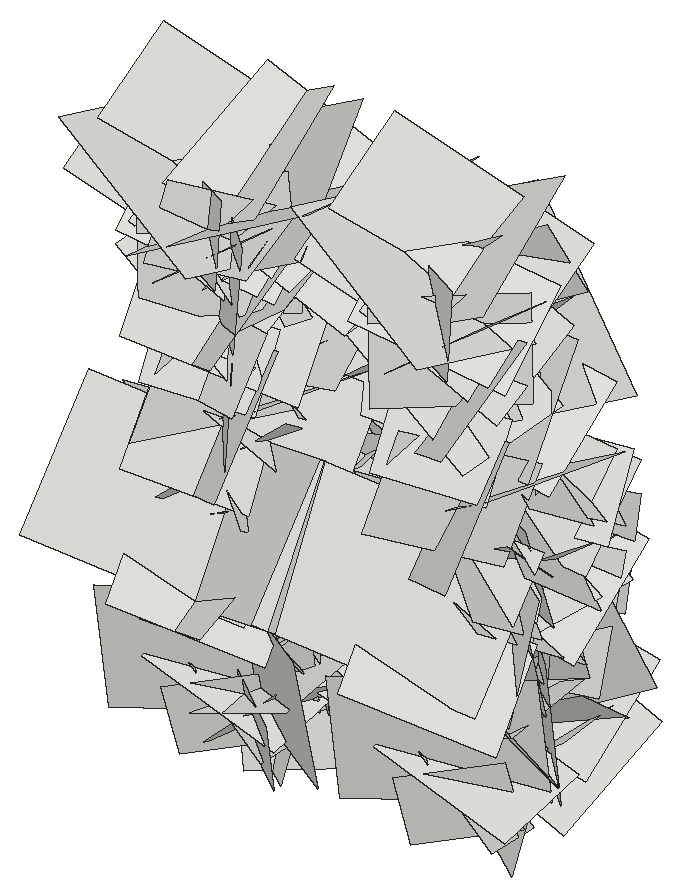
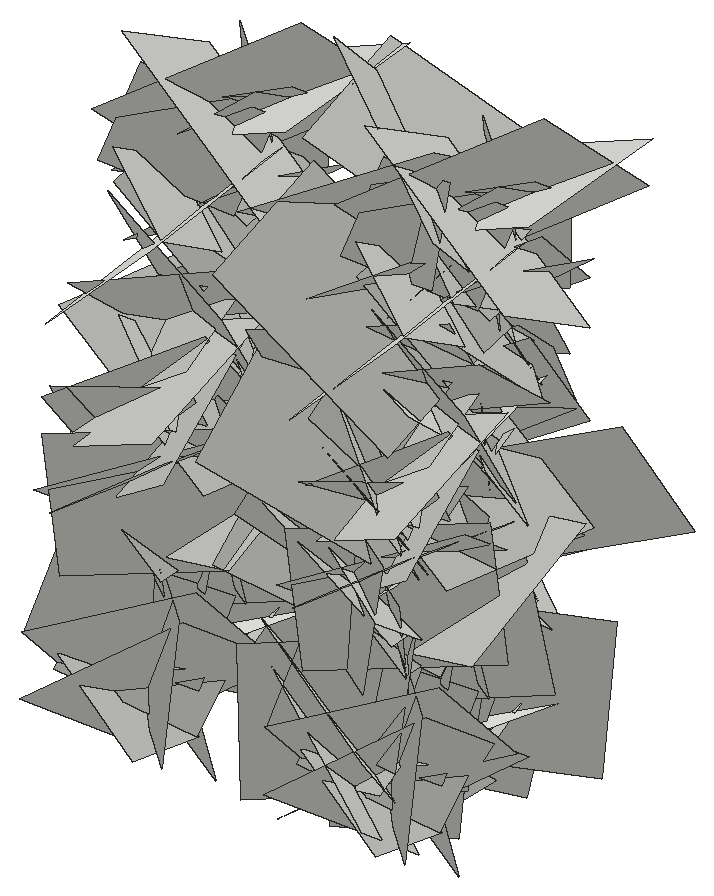
# SketchUp Ruby script. Lengths in inches.
U = 1.inch
M = Sketchup.active_model
def pt(a) = Geom::Point3d.new(a.map { |v| v * U })
def face(e, loops, mat)
  f = e.add_face(loops[0].map { |a| pt(a) })
  loops[1..].each { |l| e.add_face(l.map { |a| pt(a) }).erase! }
  f.material = f.back_material = mat if mat
  f
end
# faces: each face lists its corners as indices into pts; further lists are holes
def faces(e, pts, list, mat = nil) = list.each { |f| face(e, (f[0].is_a?(Array) ? f : [f]).map { |l| l.map { |i| pts[i] } }, mat) }
# xy, xz, yz: faces in a plane at the given z, y or x. An outline is a flat list of corners, or four numbers for a rectangle; further outlines are holes
def ring(l) = l.size == 4 ? [[l[0], l[1]], [l[2], l[1]], [l[2], l[3]], [l[0], l[3]]] : l.each_slice(2).to_a
def flat(e, list, mat, &to3) = list.each { |f| face(e, (f[0].is_a?(Array) ? f : [f]).map { |l| ring(l).map { |u, v| to3.(u, v) } }, mat) }
def xy(e, z, list, mat = nil) = flat(e, list, mat) { |x, y| [x, y, z] }
def xz(e, y, list, mat = nil) = flat(e, list, mat) { |x, z| [x, y, z] }
def yz(e, x, list, mat = nil) = flat(e, list, mat) { |y, z| [x, y, z] }
def lines(e, pts, list) = list.each { |a, b| e.add_line(pt(pts[a]), pt(pts[b])) }
# prism: a flat outline (further loops are holes) pulled along v
def prism(e, loops, v, mat = nil)
  f = face(e, loops, mat); d = Geom::Vector3d.new(v.map { |x| x * U })
  f.pushpull(f.normal.samedirection?(d) ? d.length : -d.length)
end
def box(e, o, s, mat = nil) = prism(e, [[o, [o[0] + s[0], o[1], o[2]], [o[0] + s[0], o[1] + s[1], o[2]], [o[0], o[1] + s[1], o[2]]]], [0, 0, s[2]], mat)
def at(x, y, z, deg = 0) = Geom::Transformation.translation(pt([x, y, z])) * Geom::Transformation.rotation(ORIGIN, Z_AXIS, deg.degrees)
def axes(o, x, y, z) = Geom::Transformation.new([*x, 0, *y, 0, *z, 0, *pt(o).to_a, 1])
def part(name) = M.definitions.add(name)
# library, detail: a bought-in or finely detailed component or shape, given as its bounding box
def library(name, o, s) = part(name).tap { |d| box(d.entities, o, s) }
def detail(e, o, s) = box(e.add_group.entities, o, s)
def put(e, d, t, mat = nil) = e.add_instance(d, t).tap { |i| i.material = mat if mat }
def group(e, t, mat = nil) = e.add_group.tap { |g| g.transformation = t; g.material = mat if mat }.entities
root = M.entities
c1 = part("Component\#6")
p = [[0.01,0,0],[0,3.24,4.54],[4.32,3.24,4.54],[4.33,0,0]]
faces(c1.entities,p,[[0,1,2,3]])
put(root,c1,axes([18.5,177.17,11.87],[-0.09089,-0.73345,-1.16692],[-0.11565,-1.16189,0.73831],[-1.45639,0.13804,0.0142]))
put(root,c1,axes([14.53,177.17,11.87],[0.09089,-0.73345,-1.16692],[0.11565,-1.16189,0.73831],[1.45639,0.13804,0.0142]))
put(root,c1,axes([28.31,177.17,11.87],[-0.09089,-0.73345,-1.16692],[-0.11565,-1.16189,0.73831],[-1.45639,0.13804,0.0142]))
put(root,c1,axes([14.53,171.15,7.72],[-0.19789,0.75168,0.59634],[0.00491,0.60823,-0.76521],[1.01706,0.14332,0.11972]))
put(root,c1,axes([18.5,171.15,7.72],[0.19789,0.75168,0.59634],[-0.00491,0.60823,-0.76521],[-1.01706,0.14332,0.11972]))
put(root,c1,axes([24.34,171.15,7.72],[-0.19789,0.75168,0.59634],[0.00491,0.60823,-0.76521],[1.01706,0.14332,0.11972]))
put(root,c1,axes([14.53,175.79,22.11],[0.09057,-0.18477,-0.67682],[-0.07729,-0.68047,0.17656],[0.73966,-0.04848,0.10132]))
put(root,c1,axes([18.5,175.79,22.11],[-0.09057,-0.18477,-0.67682],[0.07729,-0.68047,0.17656],[-0.73966,-0.04848,0.10132]))
put(root,c1,axes([24.34,175.79,22.11],[0.09057,-0.18477,-0.67682],[-0.07729,-0.68047,0.17656],[0.73966,-0.04848,0.10132]))
put(root,c1,axes([14.53,172.87,15.39],[-0.04258,0.36909,0.59744],[0.18529,0.58484,-0.34955],[0.72096,-0.1285,0.12512]))
put(root,c1,axes([18.5,172.87,15.39],[0.04258,0.36909,0.59744],[-0.18529,0.58484,-0.34955],[-0.72096,-0.1285,0.12512]))
put(root,c1,axes([24.34,172.87,15.39],[-0.04258,0.36909,0.59744],[0.18529,0.58484,-0.34955],[0.72096,-0.1285,0.12512]))
put(root,c1,axes([18.5,176.71,20],[-0.1716,-1.2405,0.25629],[-0.15029,0.2745,1.23906],[-1.33426,0.12862,-0.17253]))
put(root,c1,axes([14.53,176.71,20],[0.1716,-1.2405,0.25629],[0.15029,0.2745,1.23906],[1.33426,0.12862,-0.17253]))
put(root,c1,axes([28.31,176.71,20],[-0.1716,-1.2405,0.25629],[-0.15029,0.2745,1.23906],[-1.33426,0.12862,-0.17253]))
put(root,c1,axes([14.53,172.9,17.79],[-0.05847,0.04666,0.93522],[-0.13105,0.92828,-0.05361],[0.98388,0.12642,0.04844]))
put(root,c1,axes([18.5,172.9,17.79],[0.05847,0.04666,0.93522],[0.13105,0.92828,-0.05361],[-0.98388,0.12642,0.04844]))
put(root,c1,axes([24.34,172.9,17.79],[-0.05847,0.04666,0.93522],[-0.13105,0.92828,-0.05361],[0.98388,0.12642,0.04844]))
put(root,c1,axes([14.53,172.44,13.26],[0.14239,0.27787,0.83247],[-0.25689,0.82117,-0.23499],[0.89411,0.19168,-0.20009]))
put(root,c1,axes([18.5,172.44,13.26],[-0.14239,0.27787,0.83247],[0.25689,0.82117,-0.23499],[-0.89411,0.19168,-0.20009]))
put(root,c1,axes([24.34,172.44,13.26],[0.14239,0.27787,0.83247],[-0.25689,0.82117,-0.23499],[0.89411,0.19168,-0.20009]))
put(root,c1,axes([14.53,178.76,18.36],[-0.19902,-0.79911,-0.76231],[-0.1591,-0.74761,0.82067],[1.1598,-0.23968,-0.01823]))
put(root,c1,axes([18.5,178.76,18.36],[0.19902,-0.79911,-0.76231],[0.1591,-0.74761,0.82067],[-1.1598,-0.23968,-0.01823]))
put(root,c1,axes([24.34,178.76,18.36],[-0.19902,-0.79911,-0.76231],[-0.1591,-0.74761,0.82067],[1.1598,-0.23968,-0.01823]))
put(root,c1,axes([18.5,178.02,21.625],[0.10055,-0.80704,-0.57155],[-0.14009,-0.57937,0.79615],[-1.03886,0.00001,-0.16268]))
put(root,c1,axes([14.53,178.02,21.625],[-0.10055,-0.80704,-0.57155],[0.14009,-0.57937,0.79615],[1.03886,0.00001,-0.16268]))
put(root,c1,axes([28.31,178.02,21.625],[0.10055,-0.80704,-0.57155],[-0.14009,-0.57937,0.79615],[-1.03886,0.00001,-0.16268]))
put(root,c1,axes([18.5,171.875,12.53],[0.03767,0.74177,1.03266],[0.14299,1.02503,-0.74093],[-1.34014,0.13022,-0.05004]))
put(root,c1,axes([14.53,171.875,12.53],[-0.03767,0.74177,1.03266],[-0.14299,1.02503,-0.74093],[1.34014,0.13022,-0.05004]))
put(root,c1,axes([28.31,171.875,12.53],[0.03767,0.74177,1.03266],[0.14299,1.02503,-0.74093],[-1.34014,0.13022,-0.05004]))
put(root,c1,axes([14.53,176.92,18.36],[0.03591,-0.7978,0.13647],[-0.05211,0.13431,0.79737],[0.85636,0.04162,0.0428]))
put(root,c1,axes([18.5,176.92,18.36],[-0.03591,-0.7978,0.13647],[0.05211,0.13431,0.79737],[-0.85636,0.04162,0.0428]))
put(root,c1,axes([24.34,176.92,18.36],[0.03591,-0.7978,0.13647],[-0.05211,0.13431,0.79737],[0.85636,0.04162,0.0428]))
put(root,c1,axes([18.5,176.79,7.17],[-0.05072,0.23896,-1.1979],[-0.10512,-1.19562,-0.23454],[-1.29052,0.088,0.06618]))
put(root,c1,axes([14.53,176.79,7.17],[0.05072,0.23896,-1.1979],[0.10512,-1.19562,-0.23454],[1.29052,0.088,0.06618]))
put(root,c1,axes([28.31,176.79,7.17],[-0.05072,0.23896,-1.1979],[-0.10512,-1.19562,-0.23454],[-1.29052,0.088,0.06618]))
put(root,c1,axes([14.53,175.07,0.3],[-0.05353,-0.16234,0.63718],[-0.01427,0.63917,0.16178],[0.69684,0.00062,0.05226]))
put(root,c1,axes([18.5,175.07,0.3],[0.05353,-0.16234,0.63718],[0.01427,0.63917,0.16178],[-0.69684,0.00062,0.05226]))
put(root,c1,axes([24.34,175.07,0.3],[-0.05353,-0.16234,0.63718],[-0.01427,0.63917,0.16178],[0.69684,0.00062,0.05226]))
put(root,c1,axes([18.5,178.16,17.01],[-0.17232,-1.0163,-0.23365],[0.0611,-0.24487,1.02499],[-1.10369,0.14512,0.09322]))
put(root,c1,axes([14.53,178.16,17.01],[0.17232,-1.0163,-0.23365],[-0.0611,-0.24487,1.02499],[1.10369,0.14512,0.09322]))
put(root,c1,axes([28.31,178.16,17.01],[-0.17232,-1.0163,-0.23365],[0.0611,-0.24487,1.02499],[-1.10369,0.14512,0.09322]))
put(root,c1,axes([18.5,178.75,19.8],[-0.0392,-0.90326,-0.49419],[0.16181,-0.49385,0.89122],[-1.07932,-0.04123,0.15156]))
put(root,c1,axes([14.53,178.75,19.8],[0.0392,-0.90326,-0.49419],[-0.16181,-0.49385,0.89122],[1.07932,-0.04123,0.15156]))
put(root,c1,axes([28.31,178.75,19.8],[-0.0392,-0.90326,-0.49419],[0.16181,-0.49385,0.89122],[-1.07932,-0.04123,0.15156]))
put(root,c1,axes([14.53,174.43,8.39],[-0.03188,0.26889,0.69876],[0.00311,0.69936,-0.269],[0.79363,0.00806,0.02912]))
put(root,c1,axes([18.5,174.43,8.39],[0.03188,0.26889,0.69876],[-0.00311,0.69936,-0.269],[-0.79363,0.00806,0.02912]))
put(root,c1,axes([24.34,174.43,8.39],[-0.03188,0.26889,0.69876],[0.00311,0.69936,-0.269],[0.79363,0.00806,0.02912]))
put(root,c1,axes([18.5,179.79,22.45],[-0.18749,-0.99323,-0.93091],[0.09936,-0.94539,0.99088],[-1.43954,0.06411,0.18963]))
put(root,c1,axes([14.53,179.79,22.45],[0.18749,-0.99323,-0.93091],[-0.09936,-0.94539,0.99088],[1.43954,0.06411,0.18963]))
put(root,c1,axes([28.31,179.79,22.45],[-0.18749,-0.99323,-0.93091],[0.09936,-0.94539,0.99088],[-1.43954,0.06411,0.18963]))
put(root,c1,axes([18.5,177.03,8.61],[-0.03763,-0.79919,0.49947],[0.19388,0.48448,0.78821],[-0.97999,0.12653,0.13676]))
put(root,c1,axes([14.53,177.03,8.61],[0.03763,-0.79919,0.49947],[-0.19388,0.48448,0.78821],[0.97999,0.12653,0.13676]))
put(root,c1,axes([28.31,177.03,8.61],[-0.03763,-0.79919,0.49947],[0.19388,0.48448,0.78821],[-0.97999,0.12653,0.13676]))
put(root,c1,axes([14.53,177.03,9.04],[-0.05145,-0.49737,0.47013],[0.11624,0.45957,0.49752],[0.71609,-0.11034,-0.04698]))
put(root,c1,axes([18.5,177.03,9.04],[0.05145,-0.49737,0.47013],[-0.11624,0.45957,0.49752],[-0.71609,-0.11034,-0.04698]))
put(root,c1,axes([24.34,177.03,9.04],[-0.05145,-0.49737,0.47013],[0.11624,0.45957,0.49752],[0.71609,-0.11034,-0.04698]))
put(root,c1,axes([18.5,179.02,2.63],[0.02304,-0.93672,-0.18796],[-0.20199,-0.18848,0.91728],[-0.99236,0.01662,-0.19107]))
put(root,c1,axes([14.53,179.02,2.63],[-0.02304,-0.93672,-0.18796],[0.20199,-0.18848,0.91728],[0.99236,0.01662,-0.19107]))
put(root,c1,axes([28.31,179.02,2.63],[0.02304,-0.93672,-0.18796],[-0.20199,-0.18848,0.91728],[-0.99236,0.01662,-0.19107]))
put(root,c1,axes([14.53,175.31,3.87],[-0.17194,0.72285,-0.14796],[-0.1038,-0.17124,-0.72925],[0.77519,0.1374,-0.13047]))
put(root,c1,axes([18.5,175.31,3.87],[0.17194,0.72285,-0.14796],[0.1038,-0.17124,-0.72925],[-0.77519,0.1374,-0.13047]))
put(root,c1,axes([24.34,175.31,3.87],[-0.17194,0.72285,-0.14796],[-0.1038,-0.17124,-0.72925],[0.77519,0.1374,-0.13047]))
put(root,c1,axes([18.5,173.88,22.27],[-0.13701,1.18016,0.66561],[-0.07419,0.66193,-1.18721],[-1.4343,-0.14697,-0.00217]))
put(root,c1,axes([14.53,173.88,22.27],[0.13701,1.18016,0.66561],[0.07419,0.66193,-1.18721],[1.4343,-0.14697,-0.00217]))
put(root,c1,axes([28.31,173.88,22.27],[-0.13701,1.18016,0.66561],[-0.07419,0.66193,-1.18721],[-1.4343,-0.14697,-0.00217]))
put(root,c1,axes([18.5,175.28,5.97],[0.1544,0.17587,1.10387],[-0.02973,1.11343,-0.17369],[-1.18449,-0.00502,0.14825]))
put(root,c1,axes([14.53,175.28,5.97],[-0.1544,0.17587,1.10387],[0.02973,1.11343,-0.17369],[1.18449,-0.00502,0.14825]))
put(root,c1,axes([28.31,175.28,5.97],[0.1544,0.17587,1.10387],[-0.02973,1.11343,-0.17369],[-1.18449,-0.00502,0.14825]))
put(root,c1,axes([18.5,174.05,15.13],[0.29087,1.34123,-0.04275],[-0.1118,-0.02194,-1.36543],[-1.41802,0.27684,0.09888]))
put(root,c1,axes([14.53,174.05,15.13],[-0.29087,1.34123,-0.04275],[0.1118,-0.02194,-1.36543],[1.41802,0.27684,0.09888]))
put(root,c1,axes([28.31,174.05,15.13],[0.29087,1.34123,-0.04275],[-0.1118,-0.02194,-1.36543],[-1.41802,0.27684,0.09888]))
put(root,c1,axes([18.5,177.91,2.6],[-0.0759,-0.493,0.60539],[-0.11612,0.60826,0.48238],[-0.8194,-0.04053,-0.12444]))
put(root,c1,axes([14.53,177.91,2.6],[0.0759,-0.493,0.60539],[0.11612,0.60826,0.48238],[0.8194,-0.04053,-0.12444]))
put(root,c1,axes([28.31,177.91,2.6],[-0.0759,-0.493,0.60539],[-0.11612,0.60826,0.48238],[-0.8194,-0.04053,-0.12444]))
put(root,c1,axes([14.53,179.07,16.9375],[0.01654,-0.76992,0.15337],[-0.18248,0.14631,0.752],[0.8119,0.04857,0.16589]))
put(root,c1,axes([18.5,179.07,16.9375],[-0.01654,-0.76992,0.15337],[0.18248,0.14631,0.752],[-0.8119,0.04857,0.16589]))
put(root,c1,axes([24.34,179.07,16.9375],[0.01654,-0.76992,0.15337],[-0.18248,0.14631,0.752],[0.8119,0.04857,0.16589]))
put(root,c1,axes([18.5,177.25,5.58],[-0.00826,-0.19404,0.73725],[-0.12542,0.72866,0.19053],[-0.79831,-0.11247,-0.03756]))
put(root,c1,axes([14.53,177.25,5.58],[0.00826,-0.19404,0.73725],[0.12542,0.72866,0.19053],[0.79831,-0.11247,-0.03756]))
put(root,c1,axes([28.31,177.25,5.58],[-0.00826,-0.19404,0.73725],[-0.12542,0.72866,0.19053],[-0.79831,-0.11247,-0.03756]))
put(root,c1,axes([14.53,178.9,4.98],[-0.12785,-0.58421,0.25103],[0.01096,0.25367,0.59532],[0.67392,-0.11496,0.03794]))
put(root,c1,axes([18.5,178.9,4.98],[0.12785,-0.58421,0.25103],[-0.01096,0.25367,0.59532],[-0.67392,-0.11496,0.03794]))
put(root,c1,axes([24.34,178.9,4.98],[-0.12785,-0.58421,0.25103],[0.01096,0.25367,0.59532],[0.67392,-0.11496,0.03794]))
put(root,c1,axes([14.53,177.55,19],[-0.11507,-0.3549,0.71119],[-0.00206,0.71791,0.35796],[0.84251,-0.04671,0.09801]))
put(root,c1,axes([18.5,177.55,19],[0.11507,-0.3549,0.71119],[0.00206,0.71791,0.35796],[-0.84251,-0.04671,0.09801]))
put(root,c1,axes([24.34,177.55,19],[-0.11507,-0.3549,0.71119],[-0.00206,0.71791,0.35796],[0.84251,-0.04671,0.09801]))
put(root,c1,axes([18.5,179.43,6.59],[-0.14458,-1.15784,0.73248],[-0.20973,0.74503,1.14083],[-1.43706,0.00775,-0.24019]))
put(root,c1,axes([14.53,179.43,6.59],[0.14458,-1.15784,0.73248],[0.20973,0.74503,1.14083],[1.43706,0.00775,-0.24019]))
put(root,c1,axes([28.31,179.43,6.59],[-0.14458,-1.15784,0.73248],[-0.20973,0.74503,1.14083],[-1.43706,0.00775,-0.24019]))
put(root,c1,axes([18.5,177.67,8.79],[-0.10774,-0.22129,0.90038],[-0.20078,0.89162,0.19775],[-0.96207,-0.1613,-0.1421]))
put(root,c1,axes([14.53,177.67,8.79],[0.10774,-0.22129,0.90038],[0.20078,0.89162,0.19775],[0.96207,-0.1613,-0.1421]))
put(root,c1,axes([28.31,177.67,8.79],[-0.10774,-0.22129,0.90038],[-0.20078,0.89162,0.19775],[-0.96207,-0.1613,-0.1421]))
put(root,c1,axes([14.53,179.66,2.51],[-0.14219,-0.09473,-0.68692],[0.01318,-0.69988,0.09409],[0.73491,-0.00578,-0.13459]))
put(root,c1,axes([18.5,179.66,2.51],[0.14219,-0.09473,-0.68692],[-0.01318,-0.69988,0.09409],[-0.73491,-0.00578,-0.13459]))
put(root,c1,axes([24.34,179.66,2.51],[-0.14219,-0.09473,-0.68692],[0.01318,-0.69988,0.09409],[0.73491,-0.00578,-0.13459]))
put(root,c1,axes([14.53,180.59,3.91],[-0.10883,-0.74668,-0.23347],[0.0349,-0.23939,0.75113],[0.82853,-0.08799,-0.06231]))
put(root,c1,axes([18.5,180.59,3.91],[0.10883,-0.74668,-0.23347],[-0.0349,-0.23939,0.75113],[-0.82853,-0.08799,-0.06231]))
put(root,c1,axes([24.34,180.59,3.91],[-0.10883,-0.74668,-0.23347],[0.0349,-0.23939,0.75113],[0.82853,-0.08799,-0.06231]))
put(root,c1,axes([14.53,180.83,12.7],[-0.12371,-0.65209,-0.45157],[-0.04757,-0.45027,0.66181],[0.83942,-0.12162,-0.02905]))
put(root,c1,axes([18.5,180.83,12.7],[0.12371,-0.65209,-0.45157],[0.04757,-0.45027,0.66181],[-0.83942,-0.12162,-0.02905]))
put(root,c1,axes([24.34,180.83,12.7],[-0.12371,-0.65209,-0.45157],[-0.04757,-0.45027,0.66181],[0.83942,-0.12162,-0.02905]))
put(root,c1,axes([18.5,180.99,16.6875],[-0.01817,-0.80344,-0.66577],[-0.22863,-0.64876,0.78846],[-1.08217,0.15055,-0.1554]))
put(root,c1,axes([14.53,180.99,16.6875],[0.01817,-0.80344,-0.66577],[0.22863,-0.64876,0.78846],[1.08217,0.15055,-0.1554]))
put(root,c1,axes([28.31,180.99,16.6875],[-0.01817,-0.80344,-0.66577],[-0.22863,-0.64876,0.78846],[-1.08217,0.15055,-0.1554]))
put(root,c1,axes([18.5,176.29,14.82],[-0.00549,0.62123,1.00169],[-0.24363,0.98194,-0.61017],[-1.22543,-0.19801,0.11682]))
put(root,c1,axes([14.53,176.29,14.82],[0.00549,0.62123,1.00169],[0.24363,0.98194,-0.61017],[1.22543,-0.19801,0.11682]))
put(root,c1,axes([28.31,176.29,14.82],[-0.00549,0.62123,1.00169],[-0.24363,0.98194,-0.61017],[-1.22543,-0.19801,0.11682]))
put(root,c1,axes([14.53,178.54,4.68],[0.06155,-0.26232,0.60589],[0.0363,0.6086,0.26022],[0.69891,-0.00851,-0.06687]))
put(root,c1,axes([18.5,178.54,4.68],[-0.06155,-0.26232,0.60589],[-0.0363,0.6086,0.26022],[-0.69891,-0.00851,-0.06687]))
put(root,c1,axes([24.34,178.54,4.68],[0.06155,-0.26232,0.60589],[0.0363,0.6086,0.26022],[0.69891,-0.00851,-0.06687]))
put(root,c1,axes([18.5,179.8125,11.71],[-0.00414,-0.7832,0.49624],[0.01003,0.49619,0.78318],[-0.98275,0.00836,0.0059]))
put(root,c1,axes([28.31,179.8125,11.71],[-0.00414,-0.7832,0.49624],[0.01003,0.49619,0.78318],[-0.98275,0.00836,0.0059]))
put(root,c1,axes([14.53,179.8125,11.71],[0.00414,-0.7832,0.49624],[-0.01003,0.49619,0.78318],[0.98275,0.00836,0.0059]))
put(root,c1,axes([18.5,181.49,10.05],[-0.07357,-0.24485,-1.22332],[-0.09578,-1.221,0.24951],[-1.31896,0.10233,0.05011]))
put(root,c1,axes([14.53,181.49,10.05],[0.07357,-0.24485,-1.22332],[0.09578,-1.221,0.24951],[1.31896,0.10233,0.05011]))
put(root,c1,axes([28.31,181.49,10.05],[-0.07357,-0.24485,-1.22332],[-0.09578,-1.221,0.24951],[-1.31896,0.10233,0.05011]))
put(root,c1,axes([14.53,181.21,19.66],[-0.0984,-0.57654,-0.29954],[-0.01889,-0.30021,0.58335],[0.68843,-0.09064,-0.02681]))
put(root,c1,axes([18.5,181.21,19.66],[0.0984,-0.57654,-0.29954],[0.01889,-0.30021,0.58335],[-0.68843,-0.09064,-0.02681]))
put(root,c1,axes([24.34,181.21,19.66],[-0.0984,-0.57654,-0.29954],[-0.01889,-0.30021,0.58335],[0.68843,-0.09064,-0.02681]))
put(root,c1,axes([14.53,181.24,7.39],[-0.09835,-0.8461,0.11424],[-0.10744,0.12502,0.84359],[0.89861,-0.07766,0.11336]))
put(root,c1,axes([18.5,181.24,7.39],[0.09835,-0.8461,0.11424],[0.10744,0.12502,0.84359],[-0.89861,-0.07766,0.11336]))
put(root,c1,axes([24.34,181.24,7.39],[-0.09835,-0.8461,0.11424],[-0.10744,0.12502,0.84359],[0.89861,-0.07766,0.11336]))
put(root,c1,axes([18.5,180.26,8.26],[0.04265,-1.00211,0.75475],[0.17142,0.75298,0.99114],[-1.31872,0.06547,0.15325]))
put(root,c1,axes([14.53,180.26,8.26],[-0.04265,-1.00211,0.75475],[-0.17142,0.75298,0.99114],[1.31872,0.06547,0.15325]))
put(root,c1,axes([28.31,180.26,8.26],[0.04265,-1.00211,0.75475],[0.17142,0.75298,0.99114],[-1.31872,0.06547,0.15325]))
put(root,c1,axes([18.5,182.69,9.96],[0.0402,-0.96504,-0.67279],[-0.04089,-0.67379,0.96431],[-1.24632,-0.00902,-0.05333]))
put(root,c1,axes([14.53,182.69,9.96],[-0.0402,-0.96504,-0.67279],[0.04089,-0.67379,0.96431],[1.24632,-0.00902,-0.05333]))
put(root,c1,axes([28.31,182.69,9.96],[0.0402,-0.96504,-0.67279],[-0.04089,-0.67379,0.96431],[-1.24632,-0.00902,-0.05333]))
put(root,c1,axes([18.5,182.3,13.14],[-0.06012,-0.59744,-0.78978],[0.12867,-0.78931,0.58836],[-1.0418,-0.06301,0.11824]))
put(root,c1,axes([14.53,182.3,13.14],[0.06012,-0.59744,-0.78978],[-0.12867,-0.78931,0.58836],[1.0418,-0.06301,0.11824]))
put(root,c1,axes([28.31,182.3,13.14],[-0.06012,-0.59744,-0.78978],[0.12867,-0.78931,0.58836],[-1.0418,-0.06301,0.11824]))
put(root,c1,axes([14.53,181.23,7.68],[0.09173,-0.20092,-0.6203],[-0.07215,-0.6251,0.19298],[0.68737,-0.0388,0.10304]))
put(root,c1,axes([18.5,181.23,7.68],[-0.09173,-0.20092,-0.6203],[0.07215,-0.6251,0.19298],[-0.68737,-0.0388,0.10304]))
put(root,c1,axes([24.34,181.23,7.68],[0.09173,-0.20092,-0.6203],[-0.07215,-0.6251,0.19298],[0.68737,-0.0388,0.10304]))
put(root,c1,axes([18.5,179.12,5.58],[-0.07323,0.67973,-0.51678],[-0.08286,-0.52133,-0.67526],[-0.90131,-0.0073,0.10406]))
put(root,c1,axes([14.53,179.12,5.58],[0.07323,0.67973,-0.51678],[0.08286,-0.52133,-0.67526],[0.90131,-0.0073,0.10406]))
put(root,c1,axes([28.31,179.12,5.58],[-0.07323,0.67973,-0.51678],[-0.08286,-0.52133,-0.67526],[-0.90131,-0.0073,0.10406]))
put(root,c1,axes([18.5,181.89,8.77],[-0.15486,-1.04414,-0.08659],[0.04063,-0.0927,1.0531],[-1.10985,0.1423,0.05063]))
put(root,c1,axes([14.53,181.89,8.77],[0.15486,-1.04414,-0.08659],[-0.04063,-0.0927,1.0531],[1.10985,0.1423,0.05063]))
put(root,c1,axes([28.31,181.89,8.77],[-0.15486,-1.04414,-0.08659],[0.04063,-0.0927,1.0531],[-1.10985,0.1423,0.05063]))
put(root,c1,axes([18.5,182.08,15.67],[-0.13861,-1.35642,0.31459],[0.2886,0.28497,1.34186],[-1.44748,0.1867,0.23742]))
put(root,c1,axes([14.53,182.08,15.67],[0.13861,-1.35642,0.31459],[-0.2886,0.28497,1.34186],[1.44748,0.1867,0.23742]))
put(root,c1,axes([28.31,182.08,15.67],[-0.13861,-1.35642,0.31459],[0.2886,0.28497,1.34186],[-1.44748,0.1867,0.23742]))
put(root,c1,axes([18.5,180.69,8.55],[0.12889,0.40226,-0.91097],[0.04748,-0.91901,-0.39983],[-1.05451,0.00779,-0.12935]))
put(root,c1,axes([28.31,180.69,8.55],[0.12889,0.40226,-0.91097],[0.04748,-0.91901,-0.39983],[-1.05451,0.00779,-0.12935]))
put(root,c1,axes([14.53,180.69,8.55],[-0.12889,0.40226,-0.91097],[-0.04748,-0.91901,-0.39983],[1.05451,0.00779,-0.12935]))
put(root,c1,axes([18.5,178.03,1.86],[-0.09591,-0.07879,1.2407],[0.19288,1.22975,0.09137],[-1.3036,0.18775,-0.07776]))
put(root,c1,axes([14.53,178.03,1.86],[0.09591,-0.07879,1.2407],[-0.19288,1.22975,0.09137],[1.3036,0.18775,-0.07776]))
put(root,c1,axes([28.31,178.03,1.86],[-0.09591,-0.07879,1.2407],[0.19288,1.22975,0.09137],[-1.3036,0.18775,-0.07776]))
put(root,c1,axes([14.53,178.57,11.38],[-0.09025,0.42259,0.64735],[0.15778,0.64804,-0.40347],[0.80413,-0.07973,0.15182]))
put(root,c1,axes([18.5,178.57,11.38],[0.09025,0.42259,0.64735],[-0.15778,0.64804,-0.40347],[-0.80413,-0.07973,0.15182]))
put(root,c1,axes([24.34,178.57,11.38],[-0.09025,0.42259,0.64735],[0.15778,0.64804,-0.40347],[0.80413,-0.07973,0.15182]))
put(root,c1,axes([18.5,181.48,10.98],[-0.16941,-1.10786,0.62997],[0.04307,0.63015,1.11849],[-1.35023,0.1591,-0.04336]))
put(root,c1,axes([14.53,181.48,10.98],[0.16941,-1.10786,0.62997],[-0.04307,0.63015,1.11849],[1.35023,0.1591,-0.04336]))
put(root,c1,axes([28.31,181.48,10.98],[-0.16941,-1.10786,0.62997],[0.04307,0.63015,1.11849],[-1.35023,0.1591,-0.04336]))
put(root,c1,axes([18.5,183.39,2.71],[-0.21072,-0.93049,-0.66529],[0.0846,-0.6849,0.93407],[-1.20954,0.1142,0.18123]))
put(root,c1,axes([14.53,183.39,2.71],[0.21072,-0.93049,-0.66529],[-0.0846,-0.6849,0.93407],[1.20954,0.1142,0.18123]))
put(root,c1,axes([28.31,183.39,2.71],[-0.21072,-0.93049,-0.66529],[0.0846,-0.6849,0.93407],[-1.20954,0.1142,0.18123]))
put(root,c1,axes([18.5,182.3,11.84],[-0.17648,0.01407,-1.1199],[-0.09677,-1.12861,-0.00061],[-1.18323,0.09021,0.16708]))
put(root,c1,axes([14.53,182.3,11.84],[0.17648,0.01407,-1.1199],[0.09677,-1.12861,-0.00061],[1.18323,0.09021,0.16708]))
put(root,c1,axes([28.31,182.3,11.84],[-0.17648,0.01407,-1.1199],[-0.09677,-1.12861,-0.00061],[-1.18323,0.09021,0.16708]))
put(root,c1,axes([18.5,183.3125,5.12],[-0.15127,-0.71846,-0.81538],[-0.11003,-0.80961,0.73154],[-1.14669,0.17246,0.03737]))
put(root,c1,axes([14.53,183.3125,5.12],[0.15127,-0.71846,-0.81538],[0.11003,-0.80961,0.73154],[1.14669,0.17246,0.03737]))
put(root,c1,axes([28.31,183.3125,5.12],[-0.15127,-0.71846,-0.81538],[-0.11003,-0.80961,0.73154],[-1.14669,0.17246,0.03737]))
put(root,c1,axes([14.53,182.67,1.51],[-0.02969,-0.72745,-0.10184],[-0.03667,-0.1005,0.72735],[0.77775,-0.03251,0.03041]))
put(root,c1,axes([18.5,182.67,1.51],[0.02969,-0.72745,-0.10184],[0.03667,-0.1005,0.72735],[-0.77775,-0.03251,0.03041]))
put(root,c1,axes([24.34,182.67,1.51],[-0.02969,-0.72745,-0.10184],[-0.03667,-0.1005,0.72735],[0.77775,-0.03251,0.03041]))
